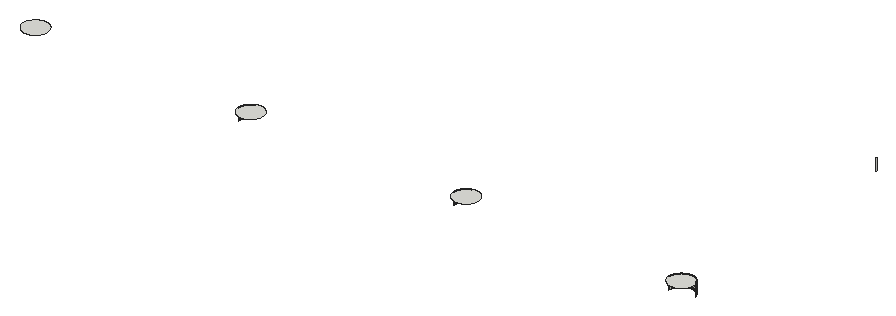
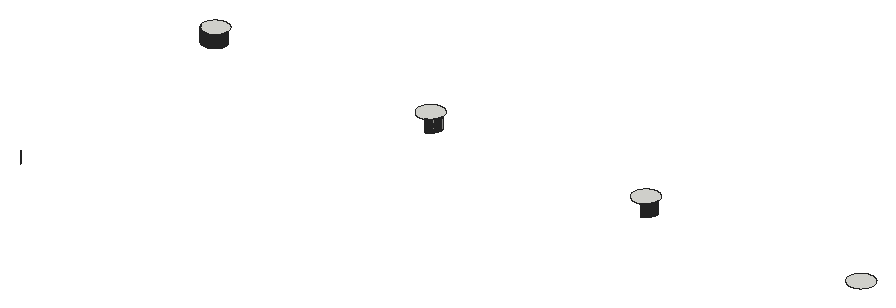
# SketchUp Ruby script. Lengths in inches.
U = 1.inch
M = Sketchup.active_model
def pt(a) = Geom::Point3d.new(a.map { |v| v * U })
def face(e, loops, mat)
  f = e.add_face(loops[0].map { |a| pt(a) })
  loops[1..].each { |l| e.add_face(l.map { |a| pt(a) }).erase! }
  f.material = f.back_material = mat if mat
  f
end
# faces: each face lists its corners as indices into pts; further lists are holes
def faces(e, pts, list, mat = nil) = list.each { |f| face(e, (f[0].is_a?(Array) ? f : [f]).map { |l| l.map { |i| pts[i] } }, mat) }
# xy, xz, yz: faces in a plane at the given z, y or x. An outline is a flat list of corners, or four numbers for a rectangle; further outlines are holes
def ring(l) = l.size == 4 ? [[l[0], l[1]], [l[2], l[1]], [l[2], l[3]], [l[0], l[3]]] : l.each_slice(2).to_a
def flat(e, list, mat, &to3) = list.each { |f| face(e, (f[0].is_a?(Array) ? f : [f]).map { |l| ring(l).map { |u, v| to3.(u, v) } }, mat) }
def xy(e, z, list, mat = nil) = flat(e, list, mat) { |x, y| [x, y, z] }
def xz(e, y, list, mat = nil) = flat(e, list, mat) { |x, z| [x, y, z] }
def yz(e, x, list, mat = nil) = flat(e, list, mat) { |y, z| [x, y, z] }
def lines(e, pts, list) = list.each { |a, b| e.add_line(pt(pts[a]), pt(pts[b])) }
# prism: a flat outline (further loops are holes) pulled along v
def prism(e, loops, v, mat = nil)
  f = face(e, loops, mat); d = Geom::Vector3d.new(v.map { |x| x * U })
  f.pushpull(f.normal.samedirection?(d) ? d.length : -d.length)
end
def box(e, o, s, mat = nil) = prism(e, [[o, [o[0] + s[0], o[1], o[2]], [o[0] + s[0], o[1] + s[1], o[2]], [o[0], o[1] + s[1], o[2]]]], [0, 0, s[2]], mat)
def at(x, y, z, deg = 0) = Geom::Transformation.translation(pt([x, y, z])) * Geom::Transformation.rotation(ORIGIN, Z_AXIS, deg.degrees)
def axes(o, x, y, z) = Geom::Transformation.new([*x, 0, *y, 0, *z, 0, *pt(o).to_a, 1])
def part(name) = M.definitions.add(name)
# library, detail: a bought-in or finely detailed component or shape, given as its bounding box
def library(name, o, s) = part(name).tap { |d| box(d.entities, o, s) }
def detail(e, o, s) = box(e.add_group.entities, o, s)
def put(e, d, t, mat = nil) = e.add_instance(d, t).tap { |i| i.material = mat if mat }
def group(e, t, mat = nil) = e.add_group.tap { |g| g.transformation = t; g.material = mat if mat }.entities
root = M.entities
xy(root,234,[[49.875,185,49.8,185.01,49.72,185.01,49.64,185.02,49.5625,185.03,49.49,185.04,49.33,185.08,49.26,185.09,49.18,185.11,49.1,185.14,49.03,185.16,48.96,185.1875,48.88,185.22,48.74,185.28,48.67,185.3125,48.6,185.35,48.53,185.39,48.46,185.42,48.39,185.47,48.33,185.51,48.26,185.55,47.96,185.8,47.79,185.97,47.59,186.21,47.55,186.27,47.5,186.34,47.46,186.4,47.34,186.61,47.31,186.68,47.27,186.75,47.21,186.89,47.18,186.97,47.16,187.04,47.13,187.12,47.11,187.19,47.09,187.27,47.07,187.34,47.06,187.42,47.04,187.5,47.03,187.58,47.02,187.65,47.01,187.73,47.01,187.81,47,187.89,47,188.125,47.01,188.2,47.01,188.28,47.02,188.36,47.03,188.4375,47.04,188.51,47.08,188.67,47.09,188.74,47.11,188.82,47.14,188.9,47.16,188.97,47.1875,189.04,47.22,189.12,47.28,189.26,47.3125,189.33,47.35,189.4,47.39,189.47,47.42,189.54,47.47,189.61,47.51,189.67,47.55,189.74,47.8,190.04,47.97,190.21,48.21,190.41,48.27,190.45,48.34,190.5,48.4,190.54,48.61,190.66,48.68,190.69,48.75,190.73,48.89,190.79,48.97,190.82,49.04,190.84,49.12,190.87,49.19,190.89,49.27,190.91,49.34,190.93,49.42,190.94,49.5,190.96,49.58,190.97,49.65,190.98,49.73,190.99,49.81,190.99,49.89,191,50.125,191,50.2,190.99,50.28,190.99,50.36,190.98,50.4375,190.97,50.51,190.96,50.67,190.92,50.74,190.91,50.82,190.89,50.9,190.86,50.97,190.84,51.04,190.8125,51.12,190.78,51.26,190.72,51.33,190.6875,51.4,190.65,51.47,190.61,51.54,190.58,51.61,190.53,51.67,190.49,51.74,190.45,52.04,190.2,52.21,190.03,52.41,189.79,52.45,189.73,52.5,189.66,52.54,189.6,52.66,189.39,52.69,189.32,52.73,189.25,52.79,189.11,52.82,189.03,52.84,188.96,52.87,188.88,52.89,188.81,52.91,188.73,52.93,188.66,52.94,188.58,52.96,188.5,52.97,188.42,52.98,188.35,52.99,188.27,52.99,188.19,53,188.11,53,187.875,52.99,187.8,52.99,187.72,52.98,187.64,52.97,187.5625,52.96,187.49,52.92,187.33,52.91,187.26,52.89,187.18,52.86,187.1,52.84,187.03,52.8125,186.96,52.78,186.88,52.72,186.74,52.6875,186.67,52.65,186.6,52.61,186.53,52.58,186.46,52.53,186.39,52.49,186.33,52.45,186.26,52.2,185.96,52.03,185.79,51.79,185.59,51.73,185.55,51.66,185.5,51.6,185.46,51.39,185.34,51.32,185.31,51.25,185.27,51.11,185.21,51.03,185.18,50.96,185.16,50.88,185.13,50.81,185.11,50.73,185.09,50.66,185.07,50.58,185.06,50.5,185.04,50.42,185.03,50.35,185.02,50.27,185.01,50.19,185.01,50.11,185],[104.68,185,104.6,185.01,104.52,185.01,104.36,185.03,104.29,185.04,104.13,185.08,104.06,185.09,103.98,185.11,103.9,185.14,103.83,185.16,103.76,185.1875,103.68,185.22,103.54,185.28,103.47,185.3125,103.4,185.35,103.33,185.39,103.26,185.42,103.19,185.47,103.13,185.51,103.0625,185.55,102.9375,185.65,102.88,185.7,102.76,185.8,102.59,185.97,102.39,186.21,102.35,186.27,102.3,186.34,102.26,186.4,102.14,186.61,102.11,186.68,102.07,186.75,102.01,186.89,101.98,186.97,101.96,187.04,101.93,187.12,101.91,187.19,101.89,187.27,101.87,187.34,101.86,187.42,101.84,187.5,101.83,187.58,101.82,187.65,101.8125,187.73,101.81,187.81,101.8,187.89,101.8,188.125,101.81,188.2,101.8125,188.28,101.82,188.36,101.83,188.4375,101.84,188.51,101.86,188.59,101.875,188.67,101.89,188.74,101.91,188.82,101.9375,188.9,101.96,188.97,101.99,189.04,102.02,189.12,102.11,189.33,102.19,189.47,102.22,189.54,102.27,189.61,102.31,189.67,102.35,189.74,102.6,190.04,102.77,190.21,103.01,190.41,103.07,190.45,103.14,190.5,103.2,190.54,103.41,190.66,103.48,190.69,103.55,190.73,103.69,190.79,103.77,190.82,103.84,190.84,103.92,190.87,103.99,190.89,104.07,190.91,104.14,190.93,104.22,190.94,104.3,190.96,104.45,190.98,104.53,190.99,104.61,190.99,104.6875,191,104.92,191,105,190.99,105.08,190.99,105.24,190.97,105.3125,190.96,105.39,190.94,105.47,190.92,105.54,190.91,105.62,190.89,105.7,190.86,105.77,190.84,105.84,190.8125,105.92,190.78,105.99,190.75,106.0625,190.72,106.13,190.6875,106.2,190.65,106.27,190.61,106.34,190.58,106.41,190.53,106.47,190.49,106.54,190.45,106.84,190.2,107.01,190.03,107.21,189.79,107.25,189.73,107.3,189.66,107.34,189.6,107.46,189.39,107.49,189.32,107.53,189.25,107.59,189.11,107.62,189.03,107.64,188.96,107.67,188.88,107.6875,188.81,107.71,188.73,107.73,188.66,107.74,188.58,107.76,188.5,107.77,188.42,107.78,188.35,107.79,188.27,107.79,188.19,107.8,188.11,107.8,187.875,107.79,187.8,107.79,187.72,107.78,187.64,107.77,187.5625,107.76,187.49,107.72,187.33,107.71,187.26,107.6875,187.18,107.66,187.1,107.64,187.03,107.61,186.96,107.58,186.88,107.49,186.67,107.41,186.53,107.375,186.46,107.33,186.39,107.29,186.33,107.25,186.26,107,185.96,106.83,185.79,106.59,185.59,106.53,185.55,106.46,185.5,106.4,185.46,106.19,185.34,106.12,185.31,106.05,185.27,105.91,185.21,105.83,185.18,105.76,185.16,105.68,185.13,105.61,185.11,105.53,185.09,105.46,185.07,105.38,185.06,105.3,185.04,105.22,185.03,105.15,185.02,105.07,185.01,104.99,185.01,104.91,185],[159.48,185,159.4,185.01,159.32,185.01,159.16,185.03,159.09,185.04,158.93,185.08,158.86,185.09,158.78,185.11,158.7,185.14,158.63,185.16,158.56,185.1875,158.48,185.22,158.34,185.28,158.27,185.3125,158.2,185.35,158.13,185.39,158.0625,185.42,157.99,185.47,157.93,185.51,157.86,185.55,157.56,185.8,157.39,185.97,157.19,186.21,157.15,186.27,157.1,186.34,157.06,186.4,156.94,186.61,156.91,186.68,156.84,186.82,156.8125,186.89,156.78,186.97,156.76,187.04,156.73,187.12,156.71,187.19,156.69,187.27,156.67,187.34,156.66,187.42,156.64,187.5,156.63,187.58,156.62,187.65,156.61,187.73,156.61,187.81,156.6,187.89,156.6,188.125,156.61,188.2,156.61,188.28,156.62,188.36,156.63,188.4375,156.64,188.51,156.68,188.67,156.69,188.74,156.71,188.82,156.74,188.9,156.76,188.97,156.79,189.04,156.82,189.12,156.91,189.33,156.99,189.47,157.02,189.54,157.07,189.61,157.11,189.67,157.15,189.74,157.4,190.04,157.57,190.21,157.625,190.26,157.75,190.36,157.81,190.41,157.875,190.45,157.9375,190.5,158,190.54,158.21,190.66,158.28,190.69,158.35,190.73,158.49,190.79,158.57,190.82,158.64,190.84,158.72,190.87,158.79,190.89,158.87,190.91,158.94,190.93,159.02,190.94,159.1,190.96,159.18,190.97,159.25,190.98,159.33,190.99,159.41,190.99,159.49,191,159.72,191,159.8,190.99,159.88,190.99,160.04,190.97,160.11,190.96,160.27,190.92,160.34,190.91,160.42,190.89,160.5,190.86,160.57,190.84,160.64,190.8125,160.72,190.78,160.86,190.72,160.93,190.6875,161,190.65,161.07,190.61,161.14,190.58,161.21,190.53,161.27,190.49,161.34,190.45,161.64,190.2,161.81,190.03,162.01,189.79,162.05,189.73,162.1,189.66,162.14,189.6,162.26,189.39,162.29,189.32,162.33,189.25,162.39,189.11,162.42,189.03,162.44,188.96,162.47,188.88,162.49,188.81,162.51,188.73,162.53,188.66,162.54,188.58,162.56,188.5,162.57,188.42,162.58,188.35,162.59,188.27,162.59,188.19,162.6,188.11,162.6,187.875,162.59,187.8,162.59,187.72,162.58,187.64,162.57,187.5625,162.56,187.49,162.52,187.33,162.51,187.26,162.49,187.18,162.46,187.1,162.4375,187.03,162.41,186.96,162.38,186.88,162.29,186.67,162.21,186.53,162.18,186.46,162.13,186.39,162.09,186.33,162.05,186.26,161.8,185.96,161.74,185.9,161.6875,185.85,161.63,185.79,161.39,185.59,161.33,185.55,161.26,185.5,161.2,185.46,161.13,185.42,161.0625,185.38,160.99,185.34,160.92,185.31,160.85,185.27,160.71,185.21,160.63,185.18,160.56,185.16,160.48,185.13,160.41,185.11,160.33,185.09,160.26,185.07,160.18,185.06,160.1,185.04,160.02,185.03,159.95,185.02,159.87,185.01,159.79,185.01,159.71,185],[214.28,185,214.2,185.01,214.12,185.01,213.96,185.03,213.89,185.04,213.73,185.08,213.66,185.09,213.58,185.11,213.5,185.14,213.43,185.16,213.36,185.1875,213.28,185.22,213.14,185.28,213.07,185.3125,213,185.35,212.93,185.39,212.86,185.42,212.79,185.47,212.73,185.51,212.66,185.55,212.36,185.8,212.19,185.97,211.99,186.21,211.95,186.27,211.9,186.34,211.86,186.4,211.74,186.61,211.71,186.68,211.67,186.75,211.61,186.89,211.58,186.97,211.56,187.04,211.53,187.12,211.51,187.19,211.49,187.27,211.47,187.34,211.46,187.42,211.44,187.5,211.43,187.58,211.42,187.65,211.41,187.73,211.41,187.81,211.4,187.89,211.4,188.125,211.41,188.2,211.41,188.28,211.42,188.36,211.43,188.4375,211.44,188.51,211.48,188.67,211.49,188.74,211.51,188.82,211.54,188.9,211.5625,188.97,211.59,189.04,211.62,189.12,211.71,189.33,211.79,189.47,211.82,189.54,211.87,189.61,211.91,189.67,211.95,189.74,212.2,190.04,212.26,190.1,212.3125,190.15,212.37,190.21,212.61,190.41,212.67,190.45,212.74,190.5,212.8,190.54,212.87,190.58,212.9375,190.62,213.01,190.66,213.08,190.69,213.15,190.73,213.29,190.79,213.37,190.82,213.44,190.84,213.52,190.87,213.59,190.89,213.67,190.91,213.74,190.93,213.82,190.94,213.9,190.96,213.98,190.97,214.05,190.98,214.13,190.99,214.21,190.99,214.29,191,214.52,191,214.6,190.99,214.68,190.99,214.84,190.97,214.91,190.96,215.07,190.92,215.14,190.91,215.22,190.89,215.3,190.86,215.37,190.84,215.44,190.8125,215.52,190.78,215.66,190.72,215.73,190.6875,215.8,190.65,215.87,190.61,215.9375,190.58,216.01,190.53,216.07,190.49,216.14,190.45,216.44,190.2,216.61,190.03,216.81,189.79,216.85,189.73,216.9,189.66,216.94,189.6,217.06,189.39,217.09,189.32,217.16,189.18,217.1875,189.11,217.22,189.03,217.24,188.96,217.27,188.88,217.29,188.81,217.31,188.73,217.33,188.66,217.34,188.58,217.36,188.5,217.37,188.42,217.38,188.35,217.39,188.27,217.39,188.19,217.4,188.11,217.4,187.875,217.39,187.8,217.39,187.72,217.38,187.64,217.37,187.5625,217.36,187.49,217.32,187.33,217.31,187.26,217.29,187.18,217.26,187.1,217.24,187.03,217.21,186.96,217.18,186.88,217.09,186.67,217.01,186.53,216.98,186.46,216.93,186.39,216.89,186.33,216.85,186.26,216.6,185.96,216.43,185.79,216.375,185.74,216.25,185.64,216.19,185.59,216.125,185.55,216.0625,185.5,216,185.46,215.79,185.34,215.72,185.31,215.65,185.27,215.51,185.21,215.43,185.18,215.36,185.16,215.28,185.13,215.21,185.11,215.13,185.09,215.06,185.07,214.98,185.06,214.9,185.04,214.82,185.03,214.75,185.02,214.67,185.01,214.59,185.01,214.51,185]])
xz(root,190.99,[[214.13,231,214.21,234],[214.6,231,214.68,234]])
xz(root,191,[[214.29,231,214.37,234],[214.37,231,214.45,234],[214.45,231,214.52,234]])
yz(root,101.8,[[187.89,231,187.97,234],[187.97,231,188.05,234],[188.05,231,188.125,234]])
yz(root,156.6,[[187.89,231,187.97,234],[187.97,231,188.05,234],[188.05,231,188.125,234]])
yz(root,156.61,[[188.2,231,188.28,234]])
yz(root,211.4,[[187.89,231,187.97,234],[187.97,231,188.05,234],[188.05,231,188.125,234]])
yz(root,211.41,[[188.2,231,188.28,234]])
p = [[101.8,188.125,231],[101.81,188.2,231],[101.81,188.2,234],[101.8,188.125,234],[156.6,188.125,231],[156.61,188.2,231],
  [156.61,188.2,234],[156.6,188.125,234],[211.4,188.125,231],[211.41,188.2,231],[211.41,188.2,234],[211.4,188.125,234],
  [101.8125,188.28,231],[101.8125,188.28,234],[101.82,188.36,231],[101.82,188.36,234],[156.61,188.28,231],[156.62,188.36,231],
  [156.62,188.36,234],[156.61,188.28,234],[211.41,188.28,231],[211.42,188.36,231],[211.42,188.36,234],[211.41,188.28,234],
  [101.83,188.4375,231],[101.83,188.4375,234],[101.84,188.51,231],[101.84,188.51,234],[156.63,188.4375,231],[156.63,188.4375,234],
  [156.64,188.51,231],[156.64,188.51,234],[211.43,188.4375,231],[211.43,188.4375,234],[211.44,188.51,231],[211.44,188.51,234],
  [101.86,188.59,231],[101.86,188.59,234],[156.66,188.59,231],[156.66,188.59,234],[211.46,188.59,231],[211.46,188.59,234],
  [101.875,188.67,231],[101.875,188.67,234],[156.68,188.67,231],[156.68,188.67,234],[211.48,188.67,231],[211.48,188.67,234],
  [101.89,188.74,231],[101.89,188.74,234],[101.91,188.82,231],[101.91,188.82,234],[156.69,188.74,231],[156.69,188.74,234],
  [156.71,188.82,231],[156.71,188.82,234],[211.49,188.74,231],[211.49,188.74,234],[211.51,188.82,231],[211.51,188.82,234],
  [101.9375,188.9,231],[101.9375,188.9,234],[156.74,188.9,231],[156.74,188.9,234],[211.54,188.9,231],[211.54,188.9,234],
  [101.96,188.97,231],[101.96,188.97,234],[156.76,188.97,231],[156.76,188.97,234],[211.5625,188.97,231],[211.5625,188.97,234],
  [217.24,188.96,231],[217.27,188.88,231],[217.27,188.88,234],[217.24,188.96,234],[101.99,189.04,231],[101.99,189.04,234],
  [102.02,189.12,231],[102.02,189.12,234],[156.79,189.04,231],[156.79,189.04,234],[156.82,189.12,231],[156.82,189.12,234],
  [211.59,189.04,231],[211.59,189.04,234],[211.62,189.12,231],[211.62,189.12,234],[217.1875,189.11,231],[217.22,189.03,231],
  [217.22,189.03,234],[217.1875,189.11,234],[102.05,189.19,231],[102.05,189.19,234],[156.85,189.19,231],[156.85,189.19,234],
  [211.65,189.19,231],[211.65,189.19,234],[217.16,189.18,231],[217.16,189.18,234],[102.08,189.26,231],[102.08,189.26,234],
  [156.88,189.26,231],[156.88,189.26,234],[211.68,189.26,231],[211.68,189.26,234],[217.125,189.25,231],[217.125,189.25,234],
  [102.11,189.33,231],[102.11,189.33,234],[102.15,189.4,231],[102.15,189.4,234],[156.91,189.33,231],[156.91,189.33,234],
  [156.95,189.4,231],[156.95,189.4,234],[211.71,189.33,231],[211.71,189.33,234],[211.75,189.4,231],[211.75,189.4,234],
  [217.06,189.39,231],[217.09,189.32,231],[217.09,189.32,234],[217.06,189.39,234],[102.19,189.47,231],[102.19,189.47,234],
  [156.99,189.47,231],[156.99,189.47,234],[211.79,189.47,231],[211.79,189.47,234],[217.02,189.46,231],[217.02,189.46,234],
  [102.22,189.54,231],[102.22,189.54,234],[102.27,189.61,231],[102.27,189.61,234],[157.02,189.54,231],[157.02,189.54,234],
  [157.07,189.61,231],[157.07,189.61,234],[211.82,189.54,231],[211.82,189.54,234],[211.87,189.61,231],[211.87,189.61,234],
  [216.94,189.6,231],[216.98,189.53,231],[216.98,189.53,234],[216.94,189.6,234],[102.31,189.67,231],[102.31,189.67,234],
  [157.11,189.67,231],[157.11,189.67,234],[211.91,189.67,231],[211.91,189.67,234],[216.9,189.66,231],[216.9,189.66,234],
  [102.35,189.74,231],[102.35,189.74,234],[102.4,189.8,231],[102.4,189.8,234],[157.15,189.74,231],[157.15,189.74,234],
  [157.2,189.8,231],[157.2,189.8,234],[211.95,189.74,231],[211.95,189.74,234],[212,189.8,231],[212,189.8,234],
  [216.81,189.79,231],[216.85,189.73,231],[216.85,189.73,234],[216.81,189.79,234],[102.45,189.86,231],[102.45,189.86,234],
  [157.25,189.86,231],[157.25,189.86,234],[212.05,189.86,231],[212.05,189.86,234],[216.76,189.85,231],[216.76,189.85,234],
  [102.5,189.92,231],[102.5,189.92,234],[102.55,189.98,231],[102.55,189.98,234],[157.3,189.92,231],[157.3,189.92,234],
  [157.35,189.98,231],[157.35,189.98,234],[212.1,189.92,231],[212.1,189.92,234],[212.15,189.98,231],[212.15,189.98,234],
  [216.66,189.97,231],[216.71,189.91,231],[216.71,189.91,234],[216.66,189.97,234],[102.6,190.04,231],[102.6,190.04,234],
  [102.66,190.1,231],[102.66,190.1,234],[157.4,190.04,231],[157.4,190.04,234],[157.46,190.1,231],[157.46,190.1,234],
  [212.2,190.04,231],[212.2,190.04,234],[212.26,190.1,231],[212.26,190.1,234],[216.55,190.09,231],[216.61,190.03,231],
  [216.61,190.03,234],[216.55,190.09,234],[102.71,190.15,231],[102.71,190.15,234],[157.51,190.15,231],[157.51,190.15,234],
  [212.3125,190.15,231],[212.3125,190.15,234],[216.44,190.2,231],[216.5,190.14,231],[216.5,190.14,234],[216.44,190.2,234],
  [102.77,190.21,231],[102.77,190.21,234],[102.83,190.26,231],[102.83,190.26,234],[157.57,190.21,231],[157.57,190.21,234],
  [157.625,190.26,231],[157.625,190.26,234],[212.37,190.21,231],[212.37,190.21,234],[212.43,190.26,231],[212.43,190.26,234],
  [216.38,190.25,231],[216.38,190.25,234],[102.89,190.31,231],[102.89,190.31,234],[102.95,190.36,231],[102.95,190.36,234],
  [157.6875,190.31,231],[157.6875,190.31,234],[157.75,190.36,231],[157.75,190.36,234],[212.49,190.31,231],[212.49,190.31,234],
  [212.55,190.36,231],[212.55,190.36,234],[216.26,190.35,231],[216.32,190.3,231],[216.32,190.3,234],[216.26,190.35,234],
  [103.01,190.41,231],[103.01,190.41,234],[103.07,190.45,231],[103.07,190.45,234],[157.81,190.41,231],[157.81,190.41,234],
  [157.875,190.45,231],[157.875,190.45,234],[212.61,190.41,231],[212.61,190.41,234],[212.67,190.45,231],[212.67,190.45,234],
  [216.07,190.49,231],[216.14,190.45,231],[216.14,190.45,234],[216.07,190.49,234],[216.2,190.4,231],[216.2,190.4,234],
  [103.14,190.5,231],[103.14,190.5,234],[103.2,190.54,231],[103.2,190.54,234],[103.27,190.58,231],[103.27,190.58,234],
  [157.9375,190.5,231],[157.9375,190.5,234],[158,190.54,231],[158,190.54,234],[158.07,190.58,231],[158.07,190.58,234],
  [212.74,190.5,231],[212.74,190.5,234],[212.8,190.54,231],[212.8,190.54,234],[212.87,190.58,231],[212.87,190.58,234],
  [215.9375,190.58,231],[216.01,190.53,231],[216.01,190.53,234],[215.9375,190.58,234],[103.34,190.62,231],[103.34,190.62,234],
  [103.41,190.66,231],[103.41,190.66,234],[158.14,190.62,231],[158.14,190.62,234],[158.21,190.66,231],[158.21,190.66,234],
  [212.9375,190.62,231],[212.9375,190.62,234],[213.01,190.66,231],[213.01,190.66,234],[215.8,190.65,231],[215.87,190.61,231],
  [215.87,190.61,234],[215.8,190.65,234],[103.48,190.69,231],[103.48,190.69,234],[103.55,190.73,231],[103.55,190.73,234],
  [103.62,190.76,231],[103.62,190.76,234],[158.28,190.69,231],[158.28,190.69,234],[158.35,190.73,231],[158.35,190.73,234],
  [158.42,190.76,231],[158.42,190.76,234],[213.08,190.69,231],[213.08,190.69,234],[213.15,190.73,231],[213.15,190.73,234],
  [213.22,190.76,231],[213.22,190.76,234],[215.59,190.75,231],[215.66,190.72,231],[215.66,190.72,234],[215.59,190.75,234],
  [215.73,190.6875,231],[215.73,190.6875,234],[103.69,190.79,231],[103.69,190.79,234],[103.77,190.82,231],[103.77,190.82,234],
  [103.84,190.84,231],[103.84,190.84,234],[103.92,190.87,231],[103.92,190.87,234],[158.49,190.79,231],[158.49,190.79,234],
  [158.57,190.82,231],[158.57,190.82,234],[158.64,190.84,231],[158.64,190.84,234],[158.72,190.87,231],[158.72,190.87,234],
  [213.29,190.79,231],[213.29,190.79,234],[213.37,190.82,231],[213.37,190.82,234],[213.44,190.84,231],[213.44,190.84,234],
  [213.52,190.87,231],[213.52,190.87,234],[215.3,190.86,231],[215.37,190.84,231],[215.37,190.84,234],[215.3,190.86,234],
  [215.44,190.8125,231],[215.44,190.8125,234],[215.52,190.78,231],[215.52,190.78,234],[213.59,190.89,231],[213.59,190.89,234],
  [213.67,190.91,231],[213.67,190.91,234],[213.74,190.93,231],[213.74,190.93,234],[213.82,190.94,231],[213.82,190.94,234],
  [213.9,190.96,231],[213.9,190.96,234],[214.91,190.96,231],[214.99,190.94,231],[214.99,190.94,234],[214.91,190.96,234],
  [215.07,190.92,231],[215.07,190.92,234],[215.14,190.91,231],[215.14,190.91,234],[215.22,190.89,231],[215.22,190.89,234],
  [213.98,190.97,231],[213.98,190.97,234],[214.05,190.98,231],[214.05,190.98,234],[214.13,190.99,231],[214.13,190.99,234],
  [214.21,190.99,231],[214.29,191,231],[214.29,191,234],[214.21,190.99,234],[214.52,191,231],[214.6,190.99,231],
  [214.6,190.99,234],[214.52,191,234],[214.68,190.99,231],[214.76,190.98,231],[214.76,190.98,234],[214.68,190.99,234],
  [214.84,190.97,231],[214.84,190.97,234],[213.5,251.14,231],[213.43,251.16,231],[213.43,251.16,234],[213.5,251.14,234]]
faces(root,p,[[0,1,2,3],[4,5,6,7],[8,9,10,11],[1,12,13,2],[12,14,15,13],[16,17,18,19],[20,21,22,23],[14,24,25,15],
  [24,26,27,25],[17,28,29,18],[28,30,31,29],[21,32,33,22],[32,34,35,33],[26,36,37,27],[30,38,39,31],[34,40,41,35],
  [36,42,43,37],[38,44,45,39],[40,46,47,41],[42,48,49,43],[48,50,51,49],[44,52,53,45],[52,54,55,53],[46,56,57,47],
  [56,58,59,57],[50,60,61,51],[54,62,63,55],[58,64,65,59],[60,66,67,61],[62,68,69,63],[64,70,71,65],[72,73,74,75],
  [66,76,77,67],[76,78,79,77],[68,80,81,69],[80,82,83,81],[70,84,85,71],[84,86,87,85],[88,89,90,91],[89,72,75,90],
  [78,92,93,79],[82,94,95,83],[86,96,97,87],[98,88,91,99],[92,100,101,93],[94,102,103,95],[96,104,105,97],[106,98,99,107],
  [100,108,109,101],[108,110,111,109],[102,112,113,103],[112,114,115,113],[104,116,117,105],[116,118,119,117],[120,121,122,123],[121,106,107,122],
  [110,124,125,111],[114,126,127,115],[118,128,129,119],[130,120,123,131],[124,132,133,125],[132,134,135,133],[126,136,137,127],[136,138,139,137],
  [128,140,141,129],[140,142,143,141],[144,145,146,147],[145,130,131,146],[134,148,149,135],[138,150,151,139],[142,152,153,143],[154,144,147,155],
  [148,156,157,149],[156,158,159,157],[150,160,161,151],[160,162,163,161],[152,164,165,153],[164,166,167,165],[168,169,170,171],[169,154,155,170],
  [158,172,173,159],[162,174,175,163],[166,176,177,167],[178,168,171,179],[172,180,181,173],[180,182,183,181],[174,184,185,175],[184,186,187,185],
  [176,188,189,177],[188,190,191,189],[192,193,194,195],[193,178,179,194],[182,196,197,183],[196,198,199,197],[186,200,201,187],[200,202,203,201],
  [190,204,205,191],[204,206,207,205],[208,209,210,211],[209,192,195,210],[198,212,213,199],[202,214,215,203],[206,216,217,207],[218,219,220,221],
  [219,208,211,220],[212,222,223,213],[222,224,225,223],[214,226,227,215],[226,228,229,227],[216,230,231,217],[230,232,233,231],[234,218,221,235],
  [224,236,237,225],[236,238,239,237],[228,240,241,229],[240,242,243,241],[232,244,245,233],[244,246,247,245],[248,249,250,251],[249,234,235,250],
  [238,252,253,239],[252,254,255,253],[242,256,257,243],[256,258,259,257],[246,260,261,247],[260,262,263,261],[264,265,266,267],[265,268,269,266],
  [268,248,251,269],[254,270,271,255],[270,272,273,271],[272,274,275,273],[258,276,277,259],[276,278,279,277],[278,280,281,279],[262,282,283,263],
  [282,284,285,283],[284,286,287,285],[288,289,290,291],[289,264,267,290],[274,292,293,275],[292,294,295,293],[280,296,297,281],[296,298,299,297],
  [286,300,301,287],[300,302,303,301],[304,305,306,307],[305,288,291,306],[294,308,309,295],[308,310,311,309],[310,312,313,311],[298,314,315,299],
  [314,316,317,315],[316,318,319,317],[302,320,321,303],[320,322,323,321],[322,324,325,323],[326,327,328,329],[327,330,331,328],[330,304,307,331],
  [312,332,333,313],[332,334,335,333],[334,336,337,335],[336,338,339,337],[318,340,341,319],[340,342,343,341],[342,344,345,343],[344,346,347,345],
  [324,348,349,325],[348,350,351,349],[350,352,353,351],[352,354,355,353],[356,357,358,359],[357,360,361,358],[360,362,363,361],[362,326,329,363],
  [354,364,365,355],[364,366,367,365],[366,368,369,367],[368,370,371,369],[370,372,373,371],[374,375,376,377],[375,378,379,376],[378,380,381,379],
  [380,382,383,381],[382,356,359,383],[372,384,385,373],[384,386,387,385],[386,388,389,387],[390,391,392,393],[394,395,396,397],[398,399,400,401],
  [399,402,403,400],[402,374,377,403],[404,405,406,407]])
